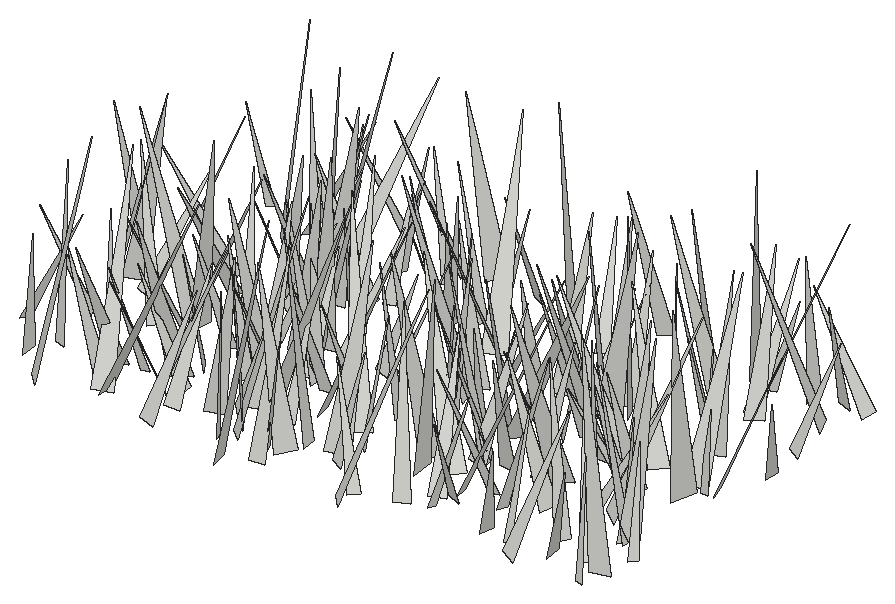
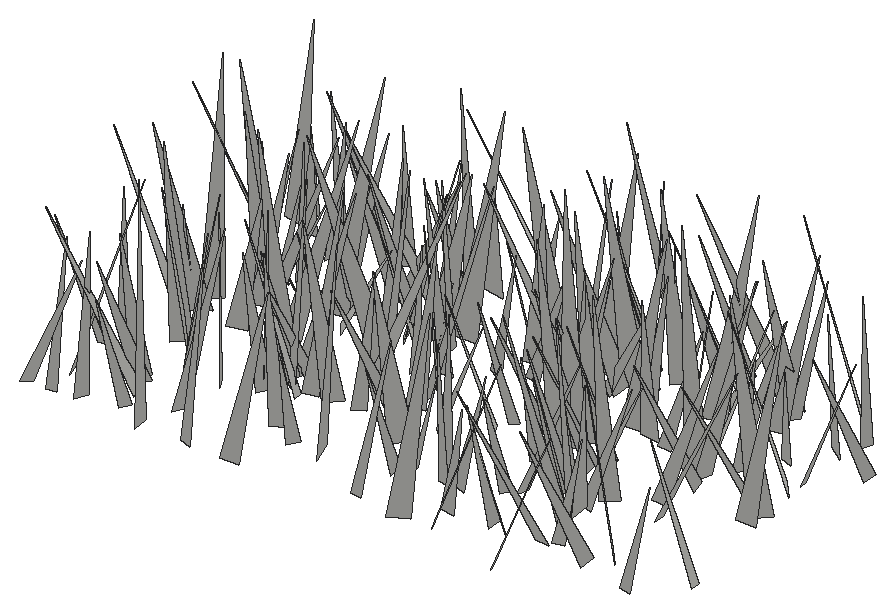
# SketchUp Ruby script. Lengths in inches.
U = 1.inch
M = Sketchup.active_model
def pt(a) = Geom::Point3d.new(a.map { |v| v * U })
def face(e, loops, mat)
  f = e.add_face(loops[0].map { |a| pt(a) })
  loops[1..].each { |l| e.add_face(l.map { |a| pt(a) }).erase! }
  f.material = f.back_material = mat if mat
  f
end
# faces: each face lists its corners as indices into pts; further lists are holes
def faces(e, pts, list, mat = nil) = list.each { |f| face(e, (f[0].is_a?(Array) ? f : [f]).map { |l| l.map { |i| pts[i] } }, mat) }
# xy, xz, yz: faces in a plane at the given z, y or x. An outline is a flat list of corners, or four numbers for a rectangle; further outlines are holes
def ring(l) = l.size == 4 ? [[l[0], l[1]], [l[2], l[1]], [l[2], l[3]], [l[0], l[3]]] : l.each_slice(2).to_a
def flat(e, list, mat, &to3) = list.each { |f| face(e, (f[0].is_a?(Array) ? f : [f]).map { |l| ring(l).map { |u, v| to3.(u, v) } }, mat) }
def xy(e, z, list, mat = nil) = flat(e, list, mat) { |x, y| [x, y, z] }
def xz(e, y, list, mat = nil) = flat(e, list, mat) { |x, z| [x, y, z] }
def yz(e, x, list, mat = nil) = flat(e, list, mat) { |y, z| [x, y, z] }
def lines(e, pts, list) = list.each { |a, b| e.add_line(pt(pts[a]), pt(pts[b])) }
# prism: a flat outline (further loops are holes) pulled along v
def prism(e, loops, v, mat = nil)
  f = face(e, loops, mat); d = Geom::Vector3d.new(v.map { |x| x * U })
  f.pushpull(f.normal.samedirection?(d) ? d.length : -d.length)
end
def box(e, o, s, mat = nil) = prism(e, [[o, [o[0] + s[0], o[1], o[2]], [o[0] + s[0], o[1] + s[1], o[2]], [o[0], o[1] + s[1], o[2]]]], [0, 0, s[2]], mat)
def at(x, y, z, deg = 0) = Geom::Transformation.translation(pt([x, y, z])) * Geom::Transformation.rotation(ORIGIN, Z_AXIS, deg.degrees)
def axes(o, x, y, z) = Geom::Transformation.new([*x, 0, *y, 0, *z, 0, *pt(o).to_a, 1])
def part(name) = M.definitions.add(name)
# library, detail: a bought-in or finely detailed component or shape, given as its bounding box
def library(name, o, s) = part(name).tap { |d| box(d.entities, o, s) }
def detail(e, o, s) = box(e.add_group.entities, o, s)
def put(e, d, t, mat = nil) = e.add_instance(d, t).tap { |i| i.material = mat if mat }
def group(e, t, mat = nil) = e.add_group.tap { |g| g.transformation = t; g.material = mat if mat }.entities
root = M.entities
c1 = part("fur_instance\#9")
p = [[0.8125,0,1.79],[0.67,-0.02,1.48],[0,-0.11,0],[0,0.11,0]]
faces(c1.entities,p,[[0,1,2,3]])
put(root,c1,axes([521.22,225.23,-21.66],[7.46967,2.68884,2.29218],[2.3982,-7.79505,1.32883],[-2.59473,0.53597,7.82688]))
put(root,c1,axes([514.8,226.19,-21.66],[0.90877,4.85728,1.17196],[4.86719,-0.59112,-1.32422],[1.13009,-1.36012,4.76083]))
put(root,c1,axes([539.5,228.57,-21.66],[4.03439,-1.67825,0.01541],[-1.64329,-3.95818,-0.85174],[-0.3411,-0.78061,4.28572]))
put(root,c1,axes([544.43,228.83,-21.66],[4.66467,-0.77947,0.02704],[-0.7406,-4.47818,-1.32848],[-0.24456,-1.30606,4.53893]))
put(root,c1,axes([522.87,227.95,-21.66],[4.02483,1.17033,1.17041],[1.40502,-4.04247,-0.78939],[-0.87491,-1.10794,4.11653]))
put(root,c1,axes([542.56,226.78,-21.66],[2.02103,5.13059,0.73898],[5.12624,-1.86067,-1.10143],[0.76856,-1.08099,5.40318]))
put(root,c1,axes([503.64,228.625,-21.66],[4.65785,-0.69082,1.21899],[-0.53967,-4.78978,-0.65231],[-1.29303,-0.48941,4.6634]))
put(root,c1,axes([547.98,227,-21.66],[1.43677,3.63281,1.03111],[3.57622,-1.66329,0.8769],[-1.21291,-0.60083,3.80693]))
put(root,c1,axes([523.82,228.53,-21.66],[4.51203,-4.20905,2.90182],[-4.30887,-5.21386,-0.8628],[-2.75143,1.26279,6.10984]))
put(root,c1,axes([509.2,228.8,-21.66],[-4.57691,0.82768,1.57562],[1.18388,4.66198,0.99001],[1.32893,-1.30255,4.54457]))
put(root,c1,axes([530.36,227.01,-21.66],[-1.14245,4.14217,0.46464],[4.01441,0.96381,1.27839],[-1.12161,-0.76952,4.10226]))
put(root,c1,axes([530.07,225.7,-21.66],[5.64336,5.1887,0.30355],[5.15395,-5.64438,0.66329],[-0.67191,0.28398,7.63742]))
put(root,c1,axes([506.14,225.98,-21.66],[-5.10797,-4.03263,5.02727],[-5.71036,5.80586,-1.14484],[2.98787,4.202,6.40647]))
put(root,c1,axes([519.36,227.5,-21.66],[-4.01098,-1.65554,1.8183],[-2.11594,4.09606,-0.93811],[1.25294,1.61753,4.23659]))
put(root,c1,axes([509.04,230.68,-21.66],[1.9027,-5.40071,0.1352],[-5.35593,-1.9045,-0.70218],[-0.70705,-0.10684,5.68285]))
put(root,c1,axes([535.49,230.35,-21.66],[-0.82646,-4.24361,0.01629],[-4.06802,0.79698,1.2278],[1.20816,-0.21938,4.14533]))
put(root,c1,axes([519.57,229.7,-21.66],[4.8829,2.83209,2.83107],[3.60518,-5.05239,-1.16384],[-1.7431,-2.51617,5.52349]))
put(root,c1,axes([510.49,227.63,-21.66],[7.61599,0.93725,0.32253],[0.89381,-7.57423,0.90437],[-0.42844,0.85927,7.61996]))
put(root,c1,axes([523.23,226.45,-21.66],[1.19903,6.87384,0.5978],[6.78552,-1.2847,1.16229],[-1.25048,-0.38022,6.88014]))
put(root,c1,axes([517.38,229.64,-21.66],[3.13574,-5.33007,1.5739],[-5.55752,-3.01682,0.85589],[-0.02918,1.79133,6.12454]))
put(root,c1,axes([548.32,228.6,-21.66],[-0.94907,-6.99906,3.73248],[-7.88487,0.42284,-1.21201],[-0.8643,3.82797,6.95835]))
put(root,c1,axes([527.21,229.29,-21.66],[1.77196,3.84512,1.4323],[4.08534,-1.50774,-1.0065],[0.38272,-1.70823,4.11239]))
put(root,c1,axes([513.53,229.63,-21.66],[-2.7685,-2.84273,0.0732],[-2.6967,2.59213,-1.32656],[-0.90237,0.97511,3.73978]))
put(root,c1,axes([512.94,231.89,-21.66],[2.89826,-6.60565,0.55734],[-6.55377,-2.94663,-0.84295],[-0.99662,0.16719,7.16407]))
put(root,c1,axes([513.47,228.77,-21.66],[4.56915,3.9518,0.34933],[3.96081,-4.51383,-0.74378],[0.22516,-0.79028,5.99505]))
put(root,c1,axes([533.29,227.99,-21.66],[-0.40472,6.25604,0.83945],[6.18781,0.22712,1.29072],[-1.24649,-0.90382,6.13481]))
put(root,c1,axes([535.0625,228.75,-21.66],[3.77133,0.16267,0.95437],[-0.10228,-3.74984,1.04331],[-0.96272,1.03561,3.6278]))
put(root,c1,axes([514.96,228.49,-21.66],[-0.69382,4.82103,0.91338],[4.82167,0.84094,-0.77604],[0.90996,-0.78004,4.80848]))
put(root,c1,axes([514.3125,230.56,-21.66],[-4.64353,0.24048,0.81476],[0.40253,4.60984,0.93348],[0.74809,-0.98772,4.55508]))
put(root,c1,axes([541.4375,228.16,-21.66],[1.45734,4.18221,0.34787],[4.02467,-1.49715,1.13854],[-1.18907,0.05834,4.28]))
put(root,c1,axes([510.81,231.07,-21.66],[-0.75955,-3.70224,0.74684],[-3.72635,0.61048,-0.76351],[-0.61539,0.87293,3.70143]))
put(root,c1,axes([510.29,227.5,-21.66],[-0.64935,7.68845,0.01437],[7.6155,0.6412,1.06165],[-1.05669,-0.10353,7.64243]))
put(root,c1,axes([546.79,229.33,-21.66],[-1.86757,4.60063,0.33127],[4.58089,1.80817,0.71369],[-0.53944,-0.57279,4.91369]))
put(root,c1,axes([524.35,230.09,-21.66],[-6.69372,-1.63538,1.73187],[-1.91789,6.76382,-1.02573],[1.41263,1.43387,6.81383]))
put(root,c1,axes([520.12,228.31,-21.66],[5.47327,5.90798,0.9862],[5.7796,-5.55993,1.23167],[-1.57262,0.12835,7.95889]))
put(root,c1,axes([526.42,230.31,-21.66],[-2.68799,6.56885,2.98447],[6.8694,3.30396,-1.08507],[2.20641,-2.2839,7.01411]))
put(root,c1,axes([518.26,230.71,-21.66],[4.16572,3.95636,0.93283],[4.06431,-4.03236,-1.04767],[0.06588,-1.40123,5.64875]))
put(root,c1,axes([531.66,232.05,-21.66],[7.52805,-0.18805,1.99939],[0.07054,-7.72753,-0.99239],[-2.00698,-0.97696,7.46472]))
put(root,c1,axes([543.89,230.49,-21.66],[-5.59826,1.4556,0.99849],[1.35798,5.67289,-0.65612],[1.12768,0.39476,5.74707]))
put(root,c1,axes([537,232.44,-21.66],[-0.83843,-4.56243,0.7415],[-4.45874,0.59959,-1.35228],[-1.2187,0.94513,4.43735]))
put(root,c1,axes([534.55,229.94,-21.66],[-3.134,4.47853,0.59876],[4.43295,3.18866,-0.64743],[0.8745,-0.1137,5.42771]))
put(root,c1,axes([504.61,230.46,-21.66],[2.34142,5.16985,1.64131],[5.10687,-2.70355,1.23051],[-1.82787,-0.93109,5.54034]))
put(root,c1,axes([519.28,231.73,-21.66],[3.63637,-5.76719,3.12725],[-6.51934,-3.57646,0.98508],[-0.73369,3.19558,6.74635]))
put(root,c1,axes([548.88,231.15,-21.66],[-3.45785,1.40655,0.59459],[1.25916,3.45892,-0.85969],[0.86397,0.58836,3.63264]))
put(root,c1,axes([531.18,233.57,-21.66],[1.42395,-7.42701,2.10024],[-7.62151,-1.69014,-0.80943],[-1.21824,1.89264,7.51884]))
put(root,c1,axes([540.77,233.04,-21.66],[4.1746,-2.61988,2.8232],[-2.37692,-5.02847,-1.15163],[-3.03059,0.33503,4.79215]))
put(root,c1,axes([500.97,231.69,-21.66],[4.26787,-0.90452,0.30078],[-0.95208,-4.11231,1.14272],[-0.04649,1.18073,4.21035]))
put(root,c1,axes([538.54,231.3,-21.66],[5.15508,0.33774,1.32609],[0.02228,-5.18864,1.23487],[-1.36825,1.188,5.01637]))
put(root,c1,axes([520.3125,233.2,-21.66],[-2.43952,-3.83837,0.4143],[-3.75379,2.24378,-1.31547],[-0.90209,1.04325,4.3536]))
put(root,c1,axes([513.32,233.69,-21.66],[-3.34648,-2.86729,1.25208],[-2.75468,3.56945,0.81158],[1.4835,0.16004,4.33146]))
put(root,c1,axes([527.27,231.78,-21.66],[2.58432,3.47984,0.90101],[3.42396,-2.72089,0.68775],[-1.09434,-0.29537,4.2796]))
put(root,c1,axes([535.36,231.22,-21.66],[6.4283,2.09347,0.22673],[2.03253,-6.35917,1.08941],[-0.55031,0.96716,6.67224]))
put(root,c1,axes([521.74,231.37,-21.66],[-3.54385,2.2292,0.7922],[1.93522,3.55225,-1.33876],[1.36083,0.75365,3.96686]))
put(root,c1,axes([503.71,234.73,-21.66],[-4.07009,-1.55263,0.42821],[-1.43545,4.0247,0.94922],[0.73043,-0.7422,4.25151]))
put(root,c1,axes([547.19,232.72,-21.66],[-5.62081,-1.07857,0.79033],[-1.22962,5.511,-1.22409],[0.52534,1.35906,5.59093]))
put(root,c1,axes([519.67,232.44,-21.66],[7.1879,-0.3196,1.18159],[-0.53762,-7.14753,1.33717],[-1.09967,1.40532,7.06966]))
put(root,c1,axes([547.17,232.83,-21.66],[-5.57842,3.33095,2.99608],[3.28064,6.29556,-0.89096],[3.05108,-0.67911,6.43585]))
put(root,c1,axes([535.6875,235.41,-21.66],[0.34868,-5.31048,0.36463],[-5.26358,-0.28954,0.81646],[0.79301,0.41316,5.25892]))
put(root,c1,axes([539.31,236.1,-21.66],[2.6009,-7.25193,0.96085],[-7.2129,-2.71231,-0.94648],[-1.21974,0.57558,7.64587]))
put(root,c1,axes([516.49,233.9375,-21.66],[0.55696,-4.64877,2.01019],[-4.98122,-0.86859,-0.62855],[-0.91614,1.89648,4.63963]))
put(root,c1,axes([524.76,234.92,-21.66],[0.09538,-4.31944,0.7575],[-4.29634,-0.24392,-0.84995],[-0.8791,0.72346,4.23607]))
put(root,c1,axes([545.83,234.18,-21.66],[-1.72893,-3.46771,1.76985],[-3.62718,2.13831,0.64633],[1.41454,1.24466,3.82053]))
put(root,c1,axes([533.6,232.77,-21.66],[-4.22823,5.63878,0.60494],[5.64653,4.11564,1.10357],[-0.52773,-1.14251,6.96102]))
put(root,c1,axes([534,235.93,-21.66],[-4.57132,-4.01454,0.83204],[-3.89365,4.6413,1.00178],[1.28384,-0.21818,6.00082]))
put(root,c1,axes([506.25,233.23,-21.66],[0.5097,3.85536,0.87755],[3.83119,-0.70034,0.85159],[-0.9777,-0.73445,3.79452]))
put(root,c1,axes([509.72,236.33,-21.66],[-3.92471,-3.72483,0.22437],[-3.66233,3.90735,0.80501],[0.71557,-0.43166,5.35067]))
put(root,c1,axes([530.95,235.07,-21.66],[5.21956,1.10973,1.69595],[1.36173,-5.39042,-0.66376],[-1.50115,-1.03121,5.29478]))
put(root,c1,axes([543.97,233.6,-21.66],[-5.50715,-0.70612,1.61288],[-1.08889,5.52799,-1.29784],[1.38358,1.53996,5.39842]))
put(root,c1,axes([516.32,235.82,-21.66],[1.47343,-6.07806,1.78682],[-6.21699,-1.74005,-0.79238],[-1.21846,1.52838,6.20371]))
put(root,c1,axes([521.0625,236,-21.66],[-0.49716,-5.04462,0.80589],[-5.07325,0.39247,-0.67299],[-0.59982,0.86174,5.02418]))
put(root,c1,axes([525.83,233.27,-21.66],[-2.86004,7.00076,0.77945],[7.00763,2.7424,1.08181],[-0.71502,-1.12544,7.48466]))
put(root,c1,axes([522.47,233.84,-21.66],[7.12948,2.21776,0.41944],[2.17259,-7.11974,0.71624],[-0.61174,0.56098,7.43203]))
put(root,c1,axes([533.8125,234.71,-21.66],[0.03547,5.69131,1.501],[5.73382,0.30561,-1.29426],[1.32938,-1.46999,5.5423]))
put(root,c1,axes([534.32,234.94,-21.66],[-6.24639,-1.28271,0.8155],[-1.43317,6.11916,-1.35263],[0.50635,1.49608,6.23162]))
put(root,c1,axes([513.14,236.58,-21.66],[0.25989,-4.12749,1.06746],[-4.12688,-0.51192,-0.97467],[-1.06982,0.97209,4.01917]))
put(root,c1,axes([538.07,235.37,-21.66],[0.29151,4.89673,1.62599],[5.06271,0.04273,-1.03633],[0.99541,-1.65136,4.79468]))
put(root,c1,axes([542.84,235.4,-21.66],[3.55975,3.91646,0.08522],[3.79537,-3.41954,-1.38552],[0.97011,-0.99289,5.10792]))
put(root,c1,axes([531.6,235.78,-21.66],[-3.37291,-1.64413,0.77782],[-1.79286,3.28135,-0.83849],[0.30629,1.10194,3.65741]))
put(root,c1,axes([509.95,237.41,-21.66],[7.47084,-2.00529,1.5784],[-1.88161,-7.62701,-0.78379],[-1.72397,-0.36551,7.69548]))
put(root,c1,axes([544.35,234.6,-21.66],[4.64022,6.0526,0.40907],[6.0581,-4.59639,-0.71102],[0.31728,-0.75645,7.59342]))
put(root,c1,axes([526.85,235.91,-21.66],[-2.00481,-4.221,2.16779],[-4.72189,1.54205,-1.3643],[-0.46899,2.51807,4.46932]))
put(root,c1,axes([542.77,238.14,-21.66],[-3.89152,-1.38284,0.09587],[-1.31779,3.77936,1.02238],[0.42995,-0.93252,4.00136]))
put(root,c1,axes([543.67,238.125,-21.66],[3.33283,-3.55166,1.19436],[-3.37517,-3.53973,-1.10774],[-1.62758,0.06765,4.74288]))
put(root,c1,axes([533.24,235.75,-21.66],[3.40494,2.47984,0.75094],[2.39973,-3.48584,0.63038],[-0.97714,0.08048,4.16483]))
put(root,c1,axes([542.47,238.05,-21.66],[-3.58815,0.95471,1.93369],[1.59157,3.70529,1.12394],[1.45517,-1.69849,3.5388]))
put(root,c1,axes([519.88,236.48,-21.66],[-5.84783,-0.54956,0.92386],[-0.66437,5.86496,-0.71656],[0.84507,0.80798,5.82972]))
put(root,c1,axes([537.84,237.3125,-21.66],[-3.22375,-2.36609,0.00506],[-2.25529,3.0702,-1.21594],[-0.71558,0.9831,3.80952]))
put(root,c1,axes([529.29,237.74,-21.66],[-0.7765,-5.95979,2.50914],[-6.25232,1.3369,1.24057],[1.65027,2.26084,5.88073]))
put(root,c1,axes([509.01,237.98,-21.66],[-7.26017,0.65472,1.63239],[0.85,7.37598,0.82207],[1.53976,-0.9847,7.24313]))
put(root,c1,axes([507.7,235.92,-21.66],[-5.44212,1.96061,0.21811],[1.90755,5.39324,-0.88463],[0.50284,0.7598,5.71648]))
put(root,c1,axes([519.85,236.62,-21.66],[-5.54219,0.95074,1.40051],[0.80502,5.69802,-0.68242],[1.48905,0.4581,5.58158]))
put(root,c1,axes([514.65,236.0625,-21.66],[-0.46142,6.00885,1.03301],[6.04976,0.32253,0.82618],[-0.75742,-1.08443,5.96964]))
put(root,c1,axes([543.51,237.65,-21.66],[3.4619,-5.09824,2.22403],[-5.52391,-3.4582,0.67108],[-0.65172,2.22978,6.12588]))
put(root,c1,axes([546.36,239.26,-21.66],[6.94101,-3.43299,1.84422],[-3.2352,-7.17632,-1.18245],[-2.17258,-0.28153,7.65277]))
put(root,c1,axes([516.83,238.67,-21.66],[2.07554,-6.96607,1.71735],[-7.11885,-1.77704,1.39545],[0.89291,2.02467,7.13349]))
put(root,c1,axes([532.55,239.46,-21.66],[-2.91514,-5.53327,1.42514],[-5.42873,3.18122,1.24695],[1.78243,0.63944,6.12864]))
put(root,c1,axes([530.92,238.72,-21.66],[3.87563,-0.57439,1.14349],[-0.32332,-3.96837,-0.89752],[-1.23813,-0.76168,3.81378]))
put(root,c1,axes([504.06,235.8125,-21.66],[5.15399,5.0376,1.12923],[4.93282,-5.27609,1.02292],[-1.5231,-0.04087,7.13405]))
put(root,c1,axes([519.14,236.61,-21.66],[-2.23012,3.65012,0.738],[3.54975,2.34365,-0.86487],[1.12574,-0.15918,4.18913]))
put(root,c1,axes([539.7,239.76,-21.66],[-1.24664,-7.42641,1.30497],[-7.49381,1.07378,-1.04811],[-0.83512,1.45053,7.45702]))
put(root,c1,axes([542.29,238.95,-21.66],[-7.15146,0.58689,0.88826],[0.71619,7.11549,1.06478],[0.78773,-1.14116,7.09606]))
put(root,c1,axes([533.6,238.52,-21.66],[7.07032,-2.50038,0.22823],[-2.5064,-6.98854,1.08245],[0.14815,1.09629,7.42089]))
put(root,c1,axes([517.47,240,-21.66],[3.37968,-7.43588,1.46776],[-7.57694,-3.27406,0.85991],[0.19143,1.6903,8.12251]))
put(root,c1,axes([503.16,239.64,-21.66],[4.2743,-5.66959,1.70794],[-5.91958,-4.14155,1.06631],[-0.14077,2.00854,7.01974]))
put(root,c1,axes([503.41,240.77,-21.66],[0.65749,-6.30029,1.7132],[-6.47052,-0.85883,-0.67511],[-0.87239,1.62165,6.29842]))
put(root,c1,axes([514.63,239.47,-21.66],[2.82445,3.52777,0.66946],[3.53756,-2.58781,-1.2883],[0.61561,-1.31488,4.33162]))
put(root,c1,axes([531.93,241.67,-21.66],[-4.63636,-6.55031,0.51962],[-6.56307,4.58532,-0.75728],[-0.32055,0.86066,7.9893]))
put(root,c1,axes([509.1,242.02,-21.66],[0.9036,-5.03288,0.01557],[-4.93923,-0.88981,-0.97923],[-0.96652,-0.158,5.01871]))
put(root,c1,axes([528.16,240.99,-21.66],[-7.66466,-1.90179,1.421],[-1.79066,7.78455,0.75987],[1.55871,-0.40873,7.86043]))
put(root,c1,axes([537.15,241.33,-21.66],[-0.33805,-5.61743,0.95415],[-5.65981,0.22074,-0.70569],[-0.6576,0.9879,5.58317]))
put(root,c1,axes([522.22,239.86,-21.66],[0.51441,-3.71167,1.78135],[-3.92489,0.09986,1.3415],[1.24297,1.85145,3.49879]))
put(root,c1,axes([504.625,238.62,-21.66],[1.15422,4.7345,0.08294],[4.6056,-1.10261,-1.15208],[1.10037,-0.35121,4.73502]))
put(root,c1,axes([508.52,239.08,-21.66],[4.79219,0.94532,0.41054],[0.81575,-4.67249,1.23678],[-0.62985,1.14081,4.72537]))
put(root,c1,axes([517.87,239.09,-21.66],[5.65388,1.0827,1.74004],[0.6959,-5.81697,1.3583],[-1.92762,1.07564,5.59407]))
put(root,c1,axes([527.24,240.9375,-21.66],[4.80931,3.10321,2.02961],[3.46778,-4.94111,-0.66234],[-1.31293,-1.68352,5.68513]))
put(root,c1,axes([547.49,241.15,-21.66],[5.84375,1.80801,0.13219],[1.81029,-5.79638,-0.74876],[0.09603,-0.75425,6.07105]))
put(root,c1,axes([519.3,239.94,-21.66],[0.97735,4.73028,0.44464],[4.65378,-0.86171,-1.06216],[0.95682,-0.64061,4.71196]))
put(root,c1,axes([522.7,241.07,-21.66],[4.03846,2.29721,0.25382],[2.30928,-3.98992,-0.63131],[0.09403,-0.6739,4.60302]))
put(root,c1,axes([547.07,240.35,-21.66],[1.77865,4.09096,1.0407],[3.89915,-2.02489,1.29578],[-1.61729,-0.38272,4.26855]))
put(root,c1,axes([536.0625,240.22,-21.66],[3.62964,3.56201,0.97293],[3.43547,-3.75775,0.94107],[-1.35352,0.01415,4.99765]))
put(root,c1,axes([528.16,242.1,-21.66],[1.39978,-5.30319,2.32473],[-5.64349,-1.78474,-0.67328],[-1.29585,2.04412,5.44334]))
put(root,c1,axes([542.875,241.17,-21.66],[-3.19469,4.99874,1.10839],[5.10889,3.02549,1.08057],[-0.33936,-1.5103,5.83317]))
put(root,c1,axes([507.88,243.65,-21.66],[-5.4355,-1.48683,0.1699],[-1.41481,5.31415,1.24191],[0.48767,-1.15472,5.49664]))
put(root,c1,axes([534.19,244.88,-21.66],[-0.43827,-6.52973,0.002],[-6.42899,0.43186,1.145],[1.14256,-0.07472,6.44348]))
put(root,c1,axes([513.7,242.8,-21.66],[-2.53875,-3.10556,0.31926],[-3.0835,2.42999,-0.88252],[-0.48832,0.80145,3.91291]))
put(root,c1,axes([546.03,240.78,-21.66],[-1.91497,6.86191,1.78883],[6.91485,2.21764,-1.10438],[1.57179,-1.39609,7.03799]))
put(root,c1,axes([511.66,243.72,-21.66],[2.30675,-6.01681,0.97122],[-6.03702,-2.11321,1.24701],[0.83643,1.34116,6.32203]))
put(root,c1,axes([515.02,241.48,-21.66],[4.28943,0.41298,0.87796],[0.18379,-4.25331,1.1028],[-0.95267,1.03894,4.16576]))
put(root,c1,axes([536.71,243.9,-21.66],[-1.94061,6.26278,4.61542],[7.19839,3.24975,-1.38302],[2.95087,-3.80883,6.40903]))
put(root,c1,axes([548.84,244.74,-21.66],[3.9114,-1.46291,0.01114],[-1.40736,-3.77134,-1.11157],[-0.39945,-1.03737,4.02536]))
put(root,c1,axes([516.36,244.19,-21.66],[2.79226,2.81825,2.22878],[3.51982,-2.71249,-0.9798],[-0.72174,-2.32521,3.84438]))
put(root,c1,axes([525.09,243.73,-21.66],[-2.96371,-3.18096,0.56073],[-3.21747,2.84043,-0.89238],[-0.28422,1.01488,4.25508]))
put(root,c1,axes([530.68,244.48,-21.66],[2.96444,-3.24193,0.90441],[-3.19075,-3.09049,-0.61962],[-1.07107,0.23387,4.34903]))
put(root,c1,axes([512.91,242.31,-21.66],[2.64419,5.03318,0.33977],[4.95036,-2.51506,-1.26831],[0.97076,-0.88412,5.54221]))
put(root,c1,axes([514.43,244.69,-21.66],[3.42079,-7.2545,1.9343],[-7.49487,-3.17419,1.34998],[0.44283,2.31686,7.90614]))
put(root,c1,axes([535.65,244.88,-21.66],[3.71105,4.69804,3.51461],[5.68502,-3.90755,-0.77947],[-1.45074,-3.29476,5.93598]))
put(root,c1,axes([529.1,243.16,-21.66],[4.45979,0.0367,0.09292],[0.01604,-4.35825,0.95137],[-0.0986,0.95079,4.35729]))
put(root,c1,axes([544.46,244.53,-21.66],[3.53738,-5.32848,1.99163],[-5.66565,-3.51029,0.67133],[-0.50966,2.039,6.36044]))
put(root,c1,axes([512.27,245.33,-21.66],[-0.63614,-4.28295,0.71253],[-4.25699,0.4736,-0.95381],[-0.85404,0.8295,4.22357]))
put(root,c1,axes([536.11,244.03,-21.66],[4.52049,-0.19473,1.20973],[-0.39564,-4.60837,0.73662],[-1.15967,0.81315,4.46432]))
put(root,c1,axes([535.64,242.98,-21.66],[-1.08496,4.24211,0.2137],[4.12597,1.10497,-0.98676],[1.00871,0.04308,4.26602]))
put(root,c1,axes([517.94,242.91,-21.66],[-0.8094,5.47668,0.09308],[5.43232,0.79056,0.72297],[-0.70181,-0.19701,5.48875]))
put(root,c1,axes([534.66,245.46,-21.66],[5.44749,2.02001,0.26599],[2.02291,-5.27178,-1.39377],[0.24298,-1.39796,5.64031]))
put(root,c1,axes([542.72,246.16,-21.66],[3.69815,0.46024,1.83595],[1.02421,-3.87534,-1.09159],[-1.5917,-1.42435,3.56322]))
put(root,c1,axes([532.54,244.63,-21.66],[-2.8521,5.31504,2.52319],[5.50682,3.39878,-0.93481],[2.07151,-1.71732,5.95905]))
put(root,c1,axes([542.52,246.58,-21.66],[-4.88015,-2.78524,1.52655],[-2.68194,5.11285,0.7548],[1.7015,0.07051,5.5681]))
put(root,c1,axes([544.2,244.33,-21.66],[4.62309,3.63215,1.82021],[3.50208,-4.96051,1.00367],[-2.05939,-0.28182,5.79293]))
put(root,c1,axes([516.47,246.22,-21.66],[-5.33847,-0.05884,0.40473],[-0.0096,5.31499,0.64603],[0.40887,-0.64342,5.29956]))
put(root,c1,axes([521.91,246.96,-21.66],[4.60045,-1.39498,0.802],[-1.20201,-4.59424,-1.0961],[-1.06973,-0.83684,4.68067]))
put(root,c1,axes([537.4,245.1875,-21.66],[-5.47988,-2.79163,2.54101],[-3.31815,5.69792,-0.89593],[1.79996,2.00489,6.08438]))
put(root,c1,axes([539.3,247.19,-21.66],[4.52719,2.71843,2.25301],[3.1828,-4.72799,-0.69084],[-1.52829,-1.79378,5.23527]))
put(root,c1,axes([513,245.91,-21.66],[-6.34859,-2.07949,3.15929],[-2.7531,6.77324,-1.07409],[2.59343,2.09974,6.59357]))
put(root,c1,axes([512.7,245.68,-21.66],[5.61181,2.09612,1.30854],[1.89864,-5.73587,1.04566],[-1.58152,0.55181,5.89854]))
put(root,c1,axes([536.69,246.15,-21.66],[3.58302,-2.92408,2.58959],[-3.63927,-3.77537,0.77237],[-1.41842,2.30013,4.5598]))
put(root,c1,axes([514.33,245.24,-21.66],[2.31766,5.02687,0.82298],[4.84651,-2.45447,1.34356],[-1.56781,-0.15629,5.3699]))
put(root,c1,axes([512.23,246.02,-21.66],[-5.96382,1.04535,0.88629],[0.82737,5.90096,-1.39268],[1.09259,1.23747,5.8924]))
put(root,c1,axes([517.27,246.82,-21.66],[-2.50227,2.59124,1.1484],[2.47228,2.74461,-0.80603],[1.38608,-0.21748,3.51087]))
put(root,c1,axes([521,248.32,-21.66],[-1.15878,-4.12917,1.68532],[-4.31214,1.48176,0.66553],[1.13832,1.40977,4.23673]))
put(root,c1,axes([548.17,247.72,-21.66],[1.81296,4.05322,0.9149],[4.0683,-1.5284,-1.29051],[0.84535,-1.3371,4.24853]))
put(root,c1,axes([519.85,248.29,-21.66],[-1.05409,-4.02831,1.60299],[-4.27873,0.70037,-1.05356],[-0.69957,1.78611,4.02845]))
put(root,c1,axes([526.15,245.99,-21.66],[-5.32969,5.59283,1.04722],[5.46672,5.43108,-1.18331],[1.57839,0.07463,7.63447]))
put(root,c1,axes([500.93,248.77,-21.66],[4.64757,1.11707,0.03174],[1.0994,-4.54603,-0.98676],[0.20042,-0.96672,4.67697]))
put(root,c1,axes([533.22,249.15,-21.66],[1.79677,-5.19077,1.98742],[-5.55817,-1.66844,0.66734],[0.02536,2.09632,5.45226]))
put(root,c1,axes([512.23,247.58,-21.66],[7.1658,2.76652,1.69463],[2.58302,-7.35112,1.0785],[-1.96302,0.42601,7.60521]))
put(root,c1,axes([510.76,249.92,-21.66],[1.65267,-3.08975,1.39314],[-3.11179,-1.99748,-0.7386],[-1.34319,0.82596,3.42525]))
put(root,c1,axes([523.22,248.54,-21.66],[-5.0928,-0.09663,0.30052],[-0.16718,4.94609,-1.24277],[0.26777,1.25023,4.93978]))
put(root,c1,axes([547.4375,251.5,-21.66],[-6.20771,-3.16783,0.82777],[-3.08728,6.25411,0.78157],[1.09042,-0.32718,6.92531]))
put(root,c1,axes([524.13,249.08,-21.66],[3.78689,-0.0231,1.24793],[-0.32688,-3.86581,0.92039],[-1.20458,0.97644,3.67342]))
put(root,c1,axes([539.24,251.24,-21.66],[-6.05597,0.77226,2.0179],[1.21073,6.18666,1.26588],[1.78953,-1.57224,5.97233]))
put(root,c1,axes([507.14,249,-21.66],[4.85297,5.01471,2.08252],[4.89411,-5.24941,1.23566],[-2.35199,-0.5761,6.86817]))
put(root,c1,axes([529.1,250.04,-21.66],[-7.32615,-2.19993,2.60741],[-2.57876,7.61493,-0.82074],[2.23345,1.57604,7.60517]))
put(root,c1,axes([543.68,249.48,-21.66],[3.74309,-3.05687,3.19875],[-4.02453,-4.09315,0.7978],[-1.83838,2.73658,4.76642]))
put(root,c1,axes([514.06,250.93,-21.66],[2.61371,2.45973,0.53308],[2.49517,-2.43181,-1.01309],[0.32949,-1.09634,3.44317]))
put(root,c1,axes([524.23,252.85,-21.66],[-1.58112,-4.73276,0.31075],[-4.65779,1.61119,0.83937],[0.89473,0.02406,4.91878]))
put(root,c1,axes([515.36,250.43,-21.66],[4.20313,-0.16718,1.34956],[-0.39887,-4.34286,0.70427],[-1.30006,0.79192,4.14708]))
put(root,c1,axes([518.23,252.77,-21.66],[-5.1626,-2.88411,0.4563],[-2.82641,5.16852,0.6903],[0.7333,-0.3834,5.87316]))
put(root,c1,axes([507.92,250.58,-21.66],[4.70172,-1.10111,0.26171],[-1.12934,-4.49092,1.39405],[0.07438,1.41645,4.62334]))
put(root,c1,axes([503.99,251.87,-21.66],[-0.09942,-3.58739,1.13729],[-3.70553,-0.10534,-0.65623],[-0.65715,1.13676,3.52826]))
put(root,c1,axes([518.55,251.03,-21.66],[-0.54656,4.2534,1.19948],[4.32093,0.26075,1.04426],[-0.92722,-1.29209,4.15928]))
put(root,c1,axes([531.24,250.2,-21.66],[-2.96108,3.10315,0.36366],[3.04624,2.97875,-0.6142],[0.69442,0.16515,4.24503]))
put(root,c1,axes([543.19,249.99,-21.66],[-2.46279,4.53865,0.90199],[4.34757,2.61941,-1.3098],[1.58479,-0.13272,4.99491]))
put(root,c1,axes([520.41,253.42,-21.66],[4.49335,-4.83843,2.48866],[-4.8443,-5.0271,-1.02712],[-2.47721,1.05444,6.5227]))
put(root,c1,axes([511.64,250.35,-21.66],[1.69788,6.23349,0.03172],[6.16311,-1.67374,-0.97718],[0.93461,-0.28707,6.38626]))
put(root,c1,axes([546.875,254.29,-21.66],[-0.66532,-4.77379,0.4836],[-4.67341,0.75535,1.0268],[1.0873,0.32553,4.70929]))
put(root,c1,axes([542.84,250.96,-21.66],[6.48449,2.8801,0.19854],[2.8437,-6.45643,0.78158],[-0.49773,0.63448,7.05214]))
put(root,c1,axes([536.36,254.33,-21.66],[-2.50316,-5.2047,1.47138],[-5.2002,2.76171,0.92225],[1.48721,0.89649,5.70124]))
put(root,c1,axes([532.87,254.375,-21.66],[1.51569,-5.39227,1.25729],[-5.41404,-1.71643,-0.83467],[-1.15995,0.96539,5.5387]))
put(root,c1,axes([544.9375,253.78,-21.66],[-4.81176,0.83188,2.6308],[1.27412,5.3609,0.63523],[2.44739,-1.15538,4.84165]))
put(root,c1,axes([542.14,252.98,-21.66],[2.6099,-2.39325,0.8726],[-2.54736,-2.4537,0.88934],[-0.00348,1.24593,3.42758]))
put(root,c1,axes([512.07,254.68,-21.66],[-4.07436,-2.22938,0.28557],[-2.14023,4.02883,0.91657],[0.68639,-0.67121,4.55307]))
put(root,c1,axes([539.99,254.23,-21.66],[7.38345,1.68053,2.79244],[2.22073,-7.65548,-1.26461],[-2.38543,-1.92527,7.46594]))
put(root,c1,axes([548.79,254.29,-21.66],[-4.51725,1.3418,0.80765],[1.52463,4.33149,1.33117],[0.35811,-1.51528,4.52039]))
